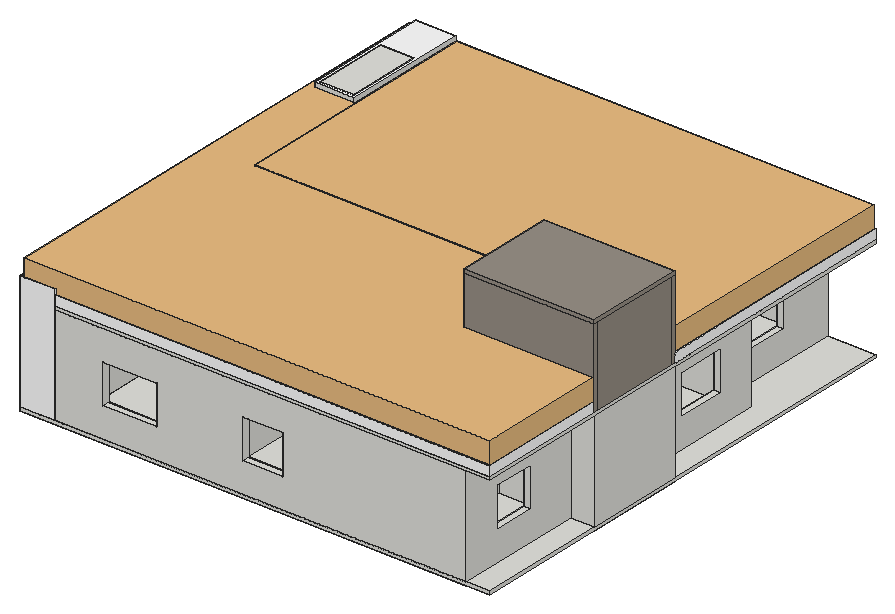
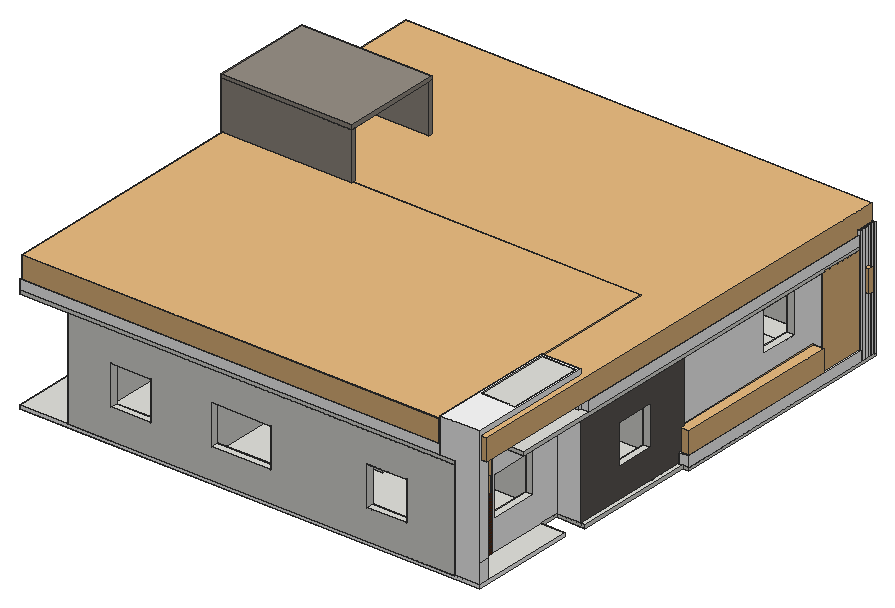
# SketchUp Ruby script. Lengths in inches.
U = 1.inch
M = Sketchup.active_model
def pt(a) = Geom::Point3d.new(a.map { |v| v * U })
def face(e, loops, mat)
  f = e.add_face(loops[0].map { |a| pt(a) })
  loops[1..].each { |l| e.add_face(l.map { |a| pt(a) }).erase! }
  f.material = f.back_material = mat if mat
  f
end
# faces: each face lists its corners as indices into pts; further lists are holes
def faces(e, pts, list, mat = nil) = list.each { |f| face(e, (f[0].is_a?(Array) ? f : [f]).map { |l| l.map { |i| pts[i] } }, mat) }
# xy, xz, yz: faces in a plane at the given z, y or x. An outline is a flat list of corners, or four numbers for a rectangle; further outlines are holes
def ring(l) = l.size == 4 ? [[l[0], l[1]], [l[2], l[1]], [l[2], l[3]], [l[0], l[3]]] : l.each_slice(2).to_a
def flat(e, list, mat, &to3) = list.each { |f| face(e, (f[0].is_a?(Array) ? f : [f]).map { |l| ring(l).map { |u, v| to3.(u, v) } }, mat) }
def xy(e, z, list, mat = nil) = flat(e, list, mat) { |x, y| [x, y, z] }
def xz(e, y, list, mat = nil) = flat(e, list, mat) { |x, z| [x, y, z] }
def yz(e, x, list, mat = nil) = flat(e, list, mat) { |y, z| [x, y, z] }
def lines(e, pts, list) = list.each { |a, b| e.add_line(pt(pts[a]), pt(pts[b])) }
# prism: a flat outline (further loops are holes) pulled along v
def prism(e, loops, v, mat = nil)
  f = face(e, loops, mat); d = Geom::Vector3d.new(v.map { |x| x * U })
  f.pushpull(f.normal.samedirection?(d) ? d.length : -d.length)
end
def box(e, o, s, mat = nil) = prism(e, [[o, [o[0] + s[0], o[1], o[2]], [o[0] + s[0], o[1] + s[1], o[2]], [o[0], o[1] + s[1], o[2]]]], [0, 0, s[2]], mat)
def at(x, y, z, deg = 0) = Geom::Transformation.translation(pt([x, y, z])) * Geom::Transformation.rotation(ORIGIN, Z_AXIS, deg.degrees)
def axes(o, x, y, z) = Geom::Transformation.new([*x, 0, *y, 0, *z, 0, *pt(o).to_a, 1])
def part(name) = M.definitions.add(name)
# library, detail: a bought-in or finely detailed component or shape, given as its bounding box
def library(name, o, s) = part(name).tap { |d| box(d.entities, o, s) }
def detail(e, o, s) = box(e.add_group.entities, o, s)
def put(e, d, t, mat = nil) = e.add_instance(d, t).tap { |i| i.material = mat if mat }
def group(e, t, mat = nil) = e.add_group.tap { |g| g.transformation = t; g.material = mat if mat }.entities
root = M.entities
M.materials.add("Bricks A03 100cm").color = [95, 90, 86]
M.materials.add("Manhattan Creative Coating MD 1125B 26.44cm").color = [255, 255, 255]
M.materials.add("Paint White Matte 002 0.02cm").color = [255, 255, 255]
M.materials.add("Pp-1846-msg 17.72cm").color = [255, 255, 255]
M.materials.add("Tiles L02 200cm").color = [152, 144, 134]
M.materials.add("Wintan - wpa36452 29.79cm").color = [255, 255, 255]
M.materials.add("Wood Mahogany 33-46 100cm").color = [84, 42, 21]
c1 = part("Stair tread")
box(c1.entities,[0,0,0],[9.89,48,7])
c2 = part("Group\#5")
box(c2.entities,[108.84,0,77],[43.96,112.5,7])
xy(c2.entities,124,[[49.47,0,59.37,48]])
xz(c2.entities,48,[[49.47,119,59.37,124]])
yz(c2.entities,49.47,[[0,119,48,124]])
put(c2.entities,c1,at(9.89,64.5,7))
put(c2.entities,c1,at(19.79,64.5,14))
put(c2.entities,c1,at(0,64.5,0))
put(c2.entities,c1,at(29.68,64.5,21))
put(c2.entities,c1,at(39.58,64.5,28))
put(c2.entities,c1,at(49.47,64.5,35))
put(c2.entities,c1,at(89.05,64.5,63))
put(c2.entities,c1,at(89.05,0,91))
put(c2.entities,c1,at(79.16,0,98))
put(c2.entities,c1,at(98.95,64.5,70))
put(c2.entities,c1,at(69.26,0,105))
put(c2.entities,c1,at(79.16,64.5,56))
put(c2.entities,c1,at(59.37,64.5,42))
put(c2.entities,c1,at(69.26,64.5,49))
put(c2.entities,c1,at(98.95,0,84))
put(c2.entities,c1,at(59.37,0,112))
c3 = part("Group\#20")
box(c3.entities,[0,0,0],[42,1.86,142.0625])
c4 = library("Group\#25",[0,0,0],[12.54,203.26,25.98])
c5 = library("Group1092\#1",[0.29,0.28,0],[3.28,6.3,0.11])
c6 = library("Group\#37",[0,0,0],[10.9375,10.44,50.62])
c7 = library("Spot Light",[-5.1,-5.1,-11.05],[10.2,10.2,11.05])
c8 = library("Group\#28",[0,0,0],[504.45,305.04,26.59])
c9 = library("Group\#27",[0,0,0],[563.06,581.04,25.98])
c10 = part("Component\#3")
xy(c10.entities,-1.4375,[[-40.6,0,0,4.4375]],"Wood Mahogany 33-46 100cm")
xy(c10.entities,3.0625,[[-40.6,0,0,4.4375]],"Wood Mahogany 33-46 100cm")
xz(c10.entities,0,[[-40.6,-1.4375,0,3.0625]],"Wood Mahogany 33-46 100cm")
xz(c10.entities,4.4375,[[-40.6,-1.4375,0,3.0625]],"Wood Mahogany 33-46 100cm")
yz(c10.entities,-40.6,[[0,-1.4375,4.4375,3.0625]],"Wood Mahogany 33-46 100cm")
yz(c10.entities,0,[[0,-1.4375,4.4375,3.0625]])
xy(root,102,[[178.31,333.5,187.31,362.5]])
xy(root,119,[[596.78,291,606.68,339]])
xy(root,120,[[[178.31,129,676.31,129,676.31,287.13,704.78,287.13,704.78,408.16,676.31,408.16,676.31,513.9,667.31,513.9,667.31,403.5,700.11,403.5,700.11,291,258.31,291,258.31,367.5,187.31,367.5,187.31,403.63,313.31,403.63,313.31,550.5,304.31,550.5,304.31,412.5,157.31,412.5,157.31,550.5,392.57,550.5,392.57,664.25,364.31,664.25,364.31,703.5,502.31,703.5,502.31,403.5,667.31,403.5,667.31,412.5,592.97,412.5,592.97,447.375,587.97,447.375,587.97,412.5,511.31,412.5,511.31,550.5,667.31,550.5,667.31,513.9,676.31,513.9,676.31,559.5,646.31,559.5,646.31,712.5,178.31,712.5,178.31,559.5,148.31,559.5,148.31,403.63,178.31,403.63],[187.31,559.5,187.31,703.5,355.31,703.5,355.31,660.44,383.57,660.44,383.57,600.44,355.31,600.44,355.31,595.72,383.57,595.72,383.57,559.5],[187.31,138,355.31,282],[511.31,138,511.31,282,587.97,282,587.97,247.1,592.97,247.1,592.97,282,667.31,282,667.31,138],[364.31,138,502.31,282],[511.31,559.5,637.31,703.5],[187.31,287,187.31,362.5,253.31,362.5,253.31,291,223.31,291,223.31,287]]])
xy(root,124,[[178.31,129,178.31,199.58,187.31,199.58,187.31,138,236.56,138,236.56,129],[236.56,129,302.56,138],[302.56,129,302.56,138,502.31,138,502.31,282,481.31,282,481.31,291,511.31,291,511.31,138,667.31,138,667.31,175.67,676.31,175.67,676.31,129],[273.14,138,273.21,138,273.27,138.01,273.34,138.02,273.4,138.03,273.46,138.05,273.52,138.08,273.58,138.1,273.64,138.13,273.7,138.17,273.85,138.29,273.97,138.44,274.01,138.5,274.04,138.56,274.0625,138.62,274.09,138.68,274.11,138.74,274.12,138.8,274.13,138.87,274.14,138.93,274.14,167.08,274.13,167.17,274.09,167.35,274.07,167.4375,274.04,167.52,273.96,167.68,273.86,167.84,273.8,167.91,273.74,167.97,273.68,168.04,273.61,168.1,273.53,168.15,273.46,168.2,273.38,168.25,273.3,168.28,273.21,168.32,273.13,168.35,272.95,168.39,272.86,168.4,272.59,168.4,272.5,168.39,272.32,168.35,272.24,168.32,272.15,168.28,272.07,168.25,271.91,168.15,271.84,168.1,271.77,168.04,271.71,167.97,271.65,167.91,271.59,167.84,271.49,167.68,271.41,167.52,271.38,167.4375,271.35,167.35,271.33,167.26,271.32,167.17,271.3125,167.08,271.31,166.99,216.79,166.99,216.79,204.56,216.98,204.5625,217.17,204.58,217.36,204.61,217.55,204.65,217.73,204.71,218.09,204.85,218.26,204.94,218.42,205.04,218.58,205.15,218.73,205.27,218.875,205.4,219.01,205.54,219.13,205.6875,219.25,205.84,219.35,206,219.45,206.17,219.53,206.34,219.6,206.52,219.66,206.7,219.71,206.89,219.75,207.08,219.77,207.27,219.78,207.46,219.78,207.65,219.77,207.84,219.75,208.04,219.71,208.22,219.66,208.41,219.6,208.59,219.53,208.77,219.45,208.94,219.35,209.11,219.25,209.27,219.13,209.43,219.01,209.57,218.875,209.71,218.73,209.84,218.58,209.96,218.42,210.07,218.26,210.17,218.09,210.26,217.91,210.34,217.55,210.46,217.36,210.5,217.17,210.53,216.98,210.55,216.79,210.56,216.79,248.125,271.31,248.125,271.3125,248.03,271.32,247.94,271.33,247.85,271.35,247.76,271.38,247.68,271.41,247.59,271.49,247.43,271.54,247.35,271.59,247.28,271.71,247.14,271.77,247.08,271.91,246.96,271.99,246.91,272.15,246.83,272.24,246.79,272.32,246.77,272.41,246.74,272.5,246.73,272.59,246.71,272.86,246.71,272.95,246.73,273.04,246.74,273.13,246.77,273.21,246.79,273.3,246.83,273.46,246.91,273.53,246.96,273.61,247.02,273.68,247.08,273.74,247.14,273.86,247.28,273.91,247.35,273.96,247.43,274.04,247.59,274.07,247.68,274.09,247.76,274.13,247.94,274.14,248.03,274.14,281.07,274.13,281.13,274.12,281.2,274.11,281.26,274.09,281.32,274.0625,281.38,274.04,281.44,274.01,281.5,273.97,281.56,273.85,281.71,273.7,281.83,273.64,281.87,273.58,281.9,273.52,281.92,273.46,281.95,273.4,281.97,273.34,281.98,273.27,281.99,273.21,282,273.14,282,355.31,282,355.31,174,364.31,174,364.31,138],[645.22,168.15,654.6,182.11,654.6,176.02,665.48,176.02,665.48,195.21,655.11,195.21,655.11,199.87,665.48,199.87,665.48,219.06,655.11,219.06,655.11,226.15,667.17,226.15,667.17,168.15],
  [355.31,174,355.31,291,334.31,286.5,313.31,291,400.31,291,400.31,287,403.31,287,403.31,286,400.31,286,400.31,282,364.31,282,364.31,174],[667.31,175.67,676.31,226.67],[654.6,182.11,654.6,182.86,655.11,182.86],[640.18,182.86,640.02,183.42,639.96,183.66,640.32,183.29,640.74,182.86],[654.6,182.86,655.11,195.21],
  [639.96,183.66,639.8,183.82,639.73,183.99,639.51,184.55,639.29,185.12,639.06,185.6875,638.83,186.25,638.6,186.82,638.37,187.38,637.89,188.5,637.14,190.15,636.88,190.68,636.61,191.22,636.34,191.74,636.0625,192.26,635.78,192.77,635.18,193.77,634.875,194.25,634.56,194.72,634.23,195.18,633.89,195.63,633.55,196.07,633.19,196.49,632.83,196.9,632.45,197.3,632.0625,197.68,631.66,198.05,631.25,198.4,630.83,198.74,630.39,199.06,629.9375,199.36,629.47,199.64,628.99,199.9,628.5,200.15,627.99,200.37,627.47,200.57,626.93,200.76,626.38,200.93,625.82,201.08,625.25,201.22,624.68,201.35,623.52,201.59,622.94,201.7,622.36,201.8,621.22,202.02,620.65,202.14,620.1,202.26,619.55,202.39,619.02,202.53,618.51,202.6875,618.01,202.86,617.53,203.04,617.07,203.25,616.63,203.47,616.22,203.72,615.83,203.99,615.46,204.29,615.11,204.6,614.79,204.94,614.49,205.29,614.21,205.67,613.94,206.0625,613.7,206.47,613.48,206.91,613.27,207.36,613.08,207.82,612.91,208.3,612.76,208.8,612.62,209.3125,612.5,209.84,612.39,210.38,612.3,210.94,612.22,211.51,612.15,212.09,612.09,212.68,612.05,213.29,612.02,213.9,611.99,214.53,611.98,215.16,611.98,215.8,611.99,216.46,612,217.11,612.02,217.78,612.05,218.46,612.13,219.82,612.17,220.51,612.23,221.21,612.28,221.91,612.34,222.61,612.4,223.32,612.47,224.02,612.53,224.73,612.67,226.15,616.25,226.15,616.22,225.53,616.1,223.64,616.01,221.78,615.99,221.16,615.97,220.55,615.95,219.9375,615.94,219.33,615.94,218.14,615.95,217.55,615.99,216.39,616.03,215.82,616.07,215.26,616.125,214.7,616.1875,214.15,616.26,213.62,616.34,213.09,616.4375,212.57,616.55,212.06,616.67,211.56,616.8,211.07,616.95,210.59,617.11,210.125,617.29,209.67,617.49,209.23,617.69,208.8,617.92,208.39,618.16,207.98,618.42,207.6,618.7,207.22,619,206.87,619.32,206.52,619.65,206.2,620.01,205.89,620.39,205.6,620.78,205.32,621.2,205.06,621.63,204.81,622.08,204.57,623.02,204.13,623.51,203.92,624,203.72,625,203.32,626.02,202.93,627.55,202.33,628.05,202.12,628.54,201.9,629.03,201.67,629.5,201.43,629.96,201.18,630.41,200.92,630.85,200.64,631.27,200.35,631.67,200.04,632.07,199.72,632.45,199.38,632.8125,199.04,633.17,198.68,633.51,198.31,633.84,197.92,634.16,197.53,634.47,197.12,634.76,196.71,635.05,196.28,635.33,195.84,635.6,195.4,635.86,194.94,636.11,194.48,636.35,194.01,636.58,193.53,636.81,193.04,637.03,192.55,637.24,192.05,637.45,191.54,637.65,191.03,637.84,190.51,638.03,189.98,638.39,188.92,638.57,188.38,638.91,187.3,639.07,186.75,639.24,186.2,639.4,185.64,639.56,185.09,639.71,184.53,639.87,183.98],[178.31,199.58,187.31,247.58],[654.6,199.87,655.11,219.06],[667.31,226.67,667.31,291,700.11,291,700.11,403.5,667.31,403.5,667.31,453.9,676.31,453.9,676.31,408.16,704.78,408.16,704.78,287.13,676.31,287.13,676.31,226.67],[178.31,247.58,178.31,333.5,187.31,333.5,187.31,287,223.31,287,223.31,291,253.31,291,253.31,330.63,258.31,330.63,258.31,291,313.31,291,313.31,282,187.31,282,187.31,247.58],
  [666.73,259.11,666.58,259.16,666.52,259.2,666.5,259.22,666.47,259.24,666.43,259.28,666.41,259.31,666.39,259.33,666.37,259.36,666.36,259.39,666.34,259.42,666.32,259.48,666.32,259.51,666.3125,259.54,666.31,259.58,666.31,269.45,667.31,269.45,667.31,259.58,667.3,259.54,667.3,259.51,667.26,259.39,667.24,259.36,667.23,259.33,667.21,259.31,667.1875,259.28,667.17,259.26,667.14,259.24,667.12,259.22,667.09,259.2,667.07,259.18,667.04,259.16,666.89,259.11],[666.31,269.45,666.31,277.78,666.3125,277.81,666.32,277.84,666.32,277.87,666.34,277.93,666.36,277.96,666.37,277.99,666.39,278.02,666.41,278.04,666.43,278.07,666.45,278.09,666.47,278.12,666.5,278.14,666.52,278.16,666.55,278.17,666.58,278.1875,666.61,278.2,666.64,278.22,666.67,278.23,666.7,278.23,666.73,278.24,666.76,278.24,666.79,278.25,666.82,278.25,666.86,278.24,666.89,278.24,666.92,278.23,666.95,278.23,666.98,278.22,667.01,278.2,667.04,278.1875,667.07,278.17,667.09,278.16,667.12,278.14,667.17,278.09,667.1875,278.07,667.21,278.04,667.23,278.02,667.24,277.99,667.26,277.96,667.3,277.84,667.3,277.81,667.31,277.78,667.31,269.45],[313.31,282,313.31,291,334.31,286.5],[313.31,282,334.31,286.5,355.31,282],[355.31,282,334.31,286.5,355.31,291],
  [400.31,282,403.31,286],[403.31,282,451.31,291],[451.31,282,451.31,291,454.31,291,454.31,287,478.31,287,478.31,291,481.31,291,481.31,282,478.31,282,478.31,286,454.31,286,454.31,282],[454.31,282,478.31,286],[400.31,287,403.31,291],
  [454.31,287,478.31,291],[304.31,291,304.31,403.5,304.43,401.96,304.43,292.54],[304.31,291,304.43,292.54,304.43,291],[304.43,291,304.43,292.54,308.81,347.25,313.31,291],[313.31,291,308.81,347.25,313.31,403.5],
  [502.31,291,502.31,291.22,502.33,291.22],[502.31,291,502.33,291.22,511.29,291.22,511.31,291],[511.31,291,511.29,291.22,511.31,291.22],[502.31,291.22,502.31,403.5,506.81,347.25,502.33,291.22],[502.33,291.22,506.81,347.25,511.29,291.22],
  [511.29,291.22,506.81,347.25,511.31,403.5,511.31,291.22],[511.31,291.22,511.37,550.5],[304.43,292.54,304.43,401.96,308.81,347.25],[178.31,333.5,178.31,367.5,258.31,367.5,258.31,362.5,187.31,362.5,187.31,333.5],[308.81,347.25,304.43,401.96,304.43,403.5,313.31,403.5],
  [506.81,347.25,502.31,403.5,511.31,403.5],[482.12,382.5,502.31,449.24],[304.43,401.96,304.31,403.5,304.31,403.63,304.43,403.63],[304.43,403.5,313.31,403.63],[547.31,403.5,547.31,412.5,587.97,412.5,587.97,447.375,592.97,447.375,592.97,412.5,667.31,412.5,667.31,403.5],
  [148.31,403.63,148.31,454.3,157.31,454.3,157.31,412.5,268.31,412.5,268.31,403.63],[268.31,403.63,268.43,412.5],[645.22,465.17,654.6,479.125,654.6,473.03,665.48,473.03,665.48,492.22,655.11,492.22,655.11,496.88,665.48,496.88,665.48,516.07,655.11,516.07,655.11,523.17,667.17,523.17,667.17,465.17],[654.6,479.125,654.6,479.87,655.11,479.87],[640.18,479.87,640.02,480.43,639.96,480.67,640.32,480.3,640.74,479.87],
  [654.6,479.87,655.11,492.22],[639.96,480.67,639.9,480.74,639.8,480.84,639.73,481,639.51,481.57,639.29,482.13,638.83,483.27,638.6,483.83,638.37,484.4,638.13,484.96,637.89,485.51,637.64,486.07,637.39,486.62,637.14,487.16,636.88,487.7,636.34,488.76,636.0625,489.27,635.78,489.78,635.48,490.29,635.18,490.78,634.875,491.26,634.56,491.73,634.23,492.2,633.89,492.65,633.55,493.08,633.19,493.51,632.83,493.92,632.45,494.32,632.0625,494.7,631.66,495.07,631.25,495.42,630.83,495.75,630.39,496.07,629.9375,496.37,629.47,496.65,628.99,496.92,628.5,497.16,627.99,497.38,627.47,497.59,626.93,497.77,626.38,497.94,625.82,498.09,625.25,498.23,624.68,498.36,623.52,498.6,622.36,498.82,620.65,499.15,619.55,499.41,619.02,499.55,618.51,499.7,618.01,499.87,617.53,500.06,617.07,500.26,616.63,500.49,616.22,500.73,615.83,501.01,615.46,501.3,615.11,501.61,614.79,501.95,614.49,502.31,614.21,502.68,613.94,503.08,613.7,503.49,613.48,503.92,613.27,504.37,613.08,504.84,612.91,505.32,612.76,505.82,612.62,506.33,612.5,506.86,612.39,507.4,612.3,507.95,612.22,508.52,612.15,509.1,612.09,509.7,612.05,510.3,612.02,510.91,611.99,511.54,611.98,512.17,611.98,512.82,611.99,513.47,612,514.13,612.02,514.8,612.05,515.47,612.09,516.15,612.17,517.53,612.23,518.22,612.28,518.92,612.4,520.33,612.47,521.04,612.53,521.75,612.67,523.17,616.25,523.17,616.22,522.54,616.14,521.28,616.1,520.66,616.07,520.03,616.01,518.79,615.99,518.18,615.97,517.5625,615.95,516.95,615.94,516.35,615.94,515.15,615.95,514.5625,615.97,513.98,615.99,513.4,616.03,512.83,616.07,512.27,616.125,511.71,616.1875,511.17,616.26,510.63,616.34,510.1,616.4375,509.58,616.55,509.07,616.67,508.57,616.8,508.08,616.95,507.6,617.11,507.14,617.29,506.68,617.49,506.24,617.69,505.81,617.92,505.4,618.16,505,618.42,504.61,618.7,504.24,619,503.88,619.32,503.54,619.65,503.21,620.01,502.9,620.39,502.61,620.78,502.33,621.2,502.07,621.63,501.82,622.08,501.59,622.55,501.36,623.02,501.14,623.51,500.94,624,500.73,624.5,500.53,625,500.34,625.51,500.14,626.02,499.95,627.04,499.55,627.55,499.34,628.05,499.13,628.54,498.91,629.03,498.6875,629.5,498.45,629.96,498.2,630.41,497.93,630.85,497.65,631.27,497.36,631.67,497.05,632.07,496.73,632.45,496.4,632.8125,496.05,633.17,495.69,633.51,495.32,633.84,494.9375,634.16,494.54,634.47,494.14,634.76,493.72,635.05,493.29,635.33,492.86,635.6,492.41,635.86,491.96,636.11,491.5,636.35,491.02,636.81,490.06,637.03,489.5625,637.24,489.0625,637.45,488.55,637.65,488.04,638.03,487,638.39,485.94,638.57,485.4,638.74,484.86,638.91,484.31,639.07,483.76,639.24,483.21,639.4,482.66,639.56,482.1,639.71,481.55,639.87,480.99],[654.6,496.88,655.11,516.07],[148.31,502.3,148.31,559.5,178.31,559.5,178.31,594.58,187.31,594.58,187.31,559.5,392.57,559.5,392.57,550.5,157.31,550.5,157.31,502.3],[392.57,550.5,502.31,559.5],
  [214.32,559.5,281.06,580.44],[637.31,586.67,646.31,646.67],[502.31,595.5,502.31,703.5,473.12,703.5,473.12,712.5,546.3125,712.5,546.3125,703.5,511.31,703.5,511.31,595.5],[355.31,595.72,355.31,600.44,383.57,600.44,383.57,660.44,355.31,660.44,355.31,703.5,284.58,703.5,284.58,712.5,401.12,712.5,401.12,703.5,364.31,703.5,364.31,664.25,392.57,664.25,392.57,595.72],[637.31,646.67,637.31,703.5,594.3125,703.5,594.3125,712.5,646.31,712.5,646.31,646.67],
  [178.31,654.58,178.31,712.5,236.58,712.5,236.58,703.5,187.31,703.5,187.31,654.58],[401.12,703.5,473.12,712.5]])
xy(root,160,[[236.56,129,302.56,138],[406.31,129,454.31,138],[667.31,175.67,676.31,226.67],[178.31,199.58,187.31,247.58],[667.31,453.9,676.31,513.9],
  [148.31,454.3,157.31,502.3],[637.31,586.67,646.31,646.67],[178.31,594.58,187.31,654.58],[236.58,703.5,284.58,712.5],[401.12,703.5,473.12,712.5],
  [546.3125,703.5,594.3125,712.5]])
xy(root,208,[[236.56,129,302.56,138],[406.31,129,454.31,138],[355.31,138,364.31,174],[667.31,175.67,676.31,226.67],[178.31,199.58,187.31,247.58],
  [403.31,282,451.31,291],[511.31,282,547.31,291],[253.31,330.63,258.31,362.5],[178.31,333.5,187.31,362.5],[178.31,367.5,187.31,403.63],
  [511.31,403.5,547.31,412.5],[268.31,403.63,304.31,412.5],[667.31,453.9,676.31,513.9],[148.31,454.3,157.31,502.3],[383.57,559.5,392.57,595.72],
  [502.31,559.5,511.31,595.5],[637.31,586.67,646.31,646.67],[178.31,594.58,187.31,654.58],[236.58,703.5,284.58,712.5],[401.12,703.5,473.12,712.5],
  [546.3125,703.5,594.3125,712.5]])
xy(root,226,[[178.31,333.5,187.31,362.5]])
xy(root,244,[[[178.31,129,676.31,129,676.31,287.13,704.78,287.13,704.78,408.16,676.31,408.16,676.31,513.9,667.31,513.9,667.31,403.5,700.11,403.5,700.11,291,258.31,291,258.31,367.5,187.31,367.5,187.31,403.63,313.31,403.63,313.31,550.5,304.31,550.5,304.31,412.5,157.31,412.5,157.31,550.5,392.57,550.5,392.57,664.25,364.31,664.25,364.31,703.5,502.31,703.5,502.31,403.5,667.31,403.5,667.31,412.5,592.97,412.5,592.97,447.375,587.97,447.375,587.97,412.5,511.31,412.5,511.31,550.5,667.31,550.5,667.31,513.9,676.31,513.9,676.31,559.5,646.31,559.5,646.31,712.5,178.31,712.5,178.31,559.5,148.31,559.5,148.31,403.63,178.31,403.63],[187.31,559.5,187.31,703.5,355.31,703.5,355.31,660.44,383.57,660.44,383.57,600.44,355.31,600.44,355.31,595.72,383.57,595.72,383.57,559.5],[187.31,138,355.31,282],[511.31,138,511.31,282,587.97,282,587.97,247.1,592.97,247.1,592.97,282,667.31,282,667.31,138],[364.31,138,502.31,282],[511.31,559.5,637.31,703.5],[187.31,287,187.31,362.5,253.31,362.5,253.31,291,223.31,291,223.31,287]]])
xy(root,290.9375,[[152.01,563.2,192.61,654.625]])
xz(root,129,[[[178.31,124,676.31,244],[236.56,160,302.56,208],[406.31,160,454.31,208]]])
xz(root,138,[[[187.31,124,187.31,244,355.31,244,355.31,208,364.31,208,364.31,244,502.31,244,502.31,124],[236.56,160,302.56,208],[406.31,160,454.31,208]],[511.31,124,667.31,244]])
xz(root,174,[[355.31,124,364.31,208]])
xz(root,175.67,[[667.31,160,676.31,208]])
xz(root,199.58,[[178.31,160,187.31,208]])
xz(root,226.67,[[667.31,160,676.31,208]])
xz(root,247.1,[[587.97,124,592.97,244]])
xz(root,247.58,[[178.31,160,187.31,208]])
xz(root,282,[[187.31,124,355.31,244],[364.31,124,403.31,124,403.31,208,451.31,208,451.31,124,502.31,124,502.31,244,364.31,244],[547.31,124,587.97,124,587.97,244,511.31,244,511.31,208,547.31,208],[592.97,124,667.31,244]])
xz(root,287,[[187.31,124,223.31,244]])
xz(root,287.13,[[676.31,124,704.78,244]])
xz(root,291,[[223.31,124,253.31,244],[258.31,124,258.31,244,700.11,244,700.11,124,547.31,124,547.31,208,511.31,208,511.31,124,451.31,124,451.31,208,403.31,208,403.31,124]])
xz(root,330.63,[[253.31,124,258.31,208]])
xz(root,333.5,[[178.31,208,187.31,226]])
xz(root,362.5,[[187.31,124,258.31,124,258.31,208,253.31,208,253.31,244,187.31,244,187.31,226,178.31,226,178.31,208,187.31,208]])
xz(root,367.5,[[178.31,124,178.31,208,187.31,208,187.31,244,258.31,244,258.31,124]])
xz(root,403.5,[[502.31,124,511.31,124,511.31,208,547.31,208,547.31,124,700.11,124,700.11,244,502.31,244]])
xz(root,403.63,[[148.31,124,268.31,124,268.31,208,304.31,208,304.31,124,313.31,124,313.31,244,187.31,244,187.31,208,178.31,208,178.31,244,148.31,244]],"Pp-1846-msg 17.72cm")
xz(root,408.16,[[676.31,124,704.78,244]])
xz(root,412.5,[[157.31,124,157.31,244,304.31,244,304.31,208,268.31,208,268.31,124],[547.31,124,547.31,208,511.31,208,511.31,244,587.97,244,587.97,124],[592.97,124,667.31,244]])
xz(root,447.375,[[587.97,124,592.97,244]])
xz(root,453.9,[[667.31,160,676.31,208]])
xz(root,454.3,[[148.31,160,157.31,208]])
xz(root,502.3,[[148.31,160,157.31,208]])
xz(root,513.9,[[667.31,160,676.31,208]])
xz(root,550.5,[[157.31,124,304.31,244],[304.31,124,313.31,244],[313.31,124,392.57,244],[511.31,124,511.37,244],[511.37,124,667.31,244]])
xz(root,559.5,[[187.31,124,187.31,244,383.57,244,383.57,208,392.57,208,392.57,124],[502.31,124,502.31,208,511.31,208,511.31,244,637.31,244,637.31,124],[646.31,124,676.31,244]])
xz(root,559.5,[[148.31,124,178.31,244]],"Pp-1846-msg 17.72cm")
xz(root,586.67,[[637.31,160,646.31,208]])
xz(root,594.58,[[178.31,160,187.31,208]])
xz(root,595.5,[[502.31,124,511.31,208]])
xz(root,595.72,[[355.31,124,392.57,124,392.57,208,383.57,208,383.57,244,355.31,244]])
xz(root,600.44,[[355.31,124,383.57,244]])
xz(root,646.67,[[637.31,160,646.31,208]])
xz(root,654.58,[[178.31,160,187.31,208]])
xz(root,660.44,[[355.31,124,383.57,244]])
xz(root,664.25,[[364.31,124,392.57,244]])
xz(root,703.5,[[[187.31,124,355.31,244],[236.58,160,284.58,208]],[[364.31,124,502.31,244],[401.12,160,473.12,208]],[511.31,124,546.3125,244],[546.3125,124,594.3125,160],[594.3125,124,637.31,124,637.31,244,546.3125,244,546.3125,208,594.3125,208]])
xz(root,712.5,[[[178.31,124,646.31,244],[401.12,160,473.12,208],[236.58,160,284.58,208],[546.3125,160,594.3125,208]]])
yz(root,148.31,[[[403.63,124,559.5,244],[454.3,160,502.3,208]]],"Bricks A03 100cm")
yz(root,157.31,[[412.5,124,454.3,124,454.3,208,502.3,208,502.3,160,454.3,160,454.3,124,550.5,124,550.5,244,412.5,244]])
yz(root,178.31,[[700.5,124,712.5,244]])
yz(root,178.31,[[[129,124,129,244,403.63,244,403.63,208,367.5,208,367.5,124],[199.58,160,247.58,208],[333.5,208,362.5,226]],[[559.5,124,700.5,244],[594.58,160,654.58,208]]],"Pp-1846-msg 17.72cm")
yz(root,187.31,[[[138,124,282,244],[199.58,160,247.58,208]],[287,124,362.5,124,362.5,208,333.5,208,333.5,226,362.5,226,362.5,244,287,244],[[559.5,124,703.5,244],[594.58,160,654.58,208]],[367.5,208,403.63,244]])
yz(root,223.31,[[287,124,291,244]])
yz(root,236.56,[[129,160,138,208]])
yz(root,236.58,[[703.5,160,712.5,208]])
yz(root,253.31,[[291,124,319.5,244],[319.5,124,319.5,244,362.5,244,362.5,208,330.63,208,330.63,124]])
yz(root,258.31,[[291,124,330.63,124,330.63,208,362.5,208,362.5,124,367.5,124,367.5,244,291,244]])
yz(root,268.31,[[403.63,124,412.5,208]])
yz(root,284.58,[[703.5,160,712.5,208]])
yz(root,302.56,[[129,160,138,208]])
yz(root,304.31,[[403.63,124,403.63,208,412.5,208,412.5,244,550.5,244,550.5,124]])
yz(root,313.31,[[403.63,124,550.5,244]])
yz(root,355.31,[[174,124,174,208,138,208,138,244,282,244,282,124],[595.72,124,600.44,244],[660.44,124,703.5,244]])
yz(root,364.31,[[174,124,282,124,282,244,138,244,138,208,174,208],[664.25,124,703.5,244]])
yz(root,383.57,[[600.44,124,660.44,244],[559.5,208,595.72,244]])
yz(root,392.57,[[550.5,124,559.5,124,559.5,208,595.72,208,595.72,124,664.25,124,664.25,244,550.5,244]])
yz(root,401.12,[[703.5,160,712.5,208]])
yz(root,403.31,[[282,124,291,208]])
yz(root,406.31,[[129,160,138,208]])
yz(root,451.31,[[282,124,291,208]])
yz(root,454.31,[[129,160,138,208]])
yz(root,473.12,[[703.5,160,712.5,208]])
yz(root,502.31,[[138,124,282,244],[403.5,124,403.5,244,703.5,244,703.5,124,595.5,124,595.5,208,559.5,208,559.5,124]])
yz(root,511.31,[[138,124,291,124,291,208,282,208,282,244,138,244],[403.5,124,550.5,124,550.5,244,412.5,244,412.5,208,403.5,208],[595.5,124,703.5,124,703.5,244,559.5,244,559.5,208,595.5,208]])
yz(root,546.3125,[[703.5,160,712.5,208]])
yz(root,547.31,[[282,124,291,208],[403.5,124,412.5,208]])
yz(root,587.97,[[247.1,124,282,244],[412.5,124,447.375,244]])
yz(root,592.97,[[247.1,124,282,244],[412.5,124,424.8,244],[424.8,124,437.1,244],[437.1,124,447.375,244]])
yz(root,594.3125,[[703.5,160,712.5,208]])
yz(root,637.31,[[[559.5,124,703.5,244],[586.67,160,646.67,208]]])
yz(root,646.31,[[[559.5,124,712.5,244],[586.67,160,646.67,208]]])
yz(root,667.31,[[[138,124,282,244],[175.67,160,226.67,208]],[412.5,124,412.5,244,513.9,244,513.9,208,453.9,208,453.9,160,513.9,160,513.9,244,550.5,244,550.5,124]])
yz(root,676.31,[[[129,124,287.13,244],[175.67,160,226.67,208]],[[408.16,124,559.5,244],[453.9,160,513.9,208]]])
yz(root,700.11,[[291,124,403.5,244]])
yz(root,704.78,[[287.13,124,408.16,244]])
g1 = group(root,at(148.31,129,120))
xy(g1,0,[[[-12,0,-12,283.19,-4.75,283.19,-4.75,430.5,30,430.5,30,454.5,0,454.5,0,583.5,556.47,583.5,556.47,0],[448.47,162,551.8,162,551.8,274.5,399,274.5,399,210,448.47,210]]],"Pp-1846-msg 17.72cm")
xy(g1,4,[[[-12,0,556.47,0,556.47,583.5,0,583.5,0,454.5,30,454.5,30,430.5,-4.75,430.5,-4.75,283.19,-12,283.19],[448.47,162,448.47,210,399,210,399,274.5,551.8,274.5,551.8,162]]])
xz(g1,0,[[-12,0,556.47,4]])
xz(g1,162,[[448.47,0,551.8,4]])
xz(g1,210,[[399,0,448.47,4]])
xz(g1,274.5,[[399,0,551.8,4]])
xz(g1,283.19,[[-12,0,-4.75,4]])
xz(g1,430.5,[[-4.75,0,0,4],[0,0,30,4]])
xz(g1,454.5,[[0,0,30,4]])
xz(g1,583.5,[[0,0,556.47,4]],"Pp-1846-msg 17.72cm")
yz(g1,-12,[[0,0,283.19,4]])
yz(g1,-4.75,[[283.19,0,430.5,4]])
yz(g1,0,[[454.5,0,583.5,4]],"Wintan - wpa36452 29.79cm")
yz(g1,30,[[430.5,0,454.5,4]])
yz(g1,399,[[210,0,274.5,4]])
yz(g1,448.47,[[162,0,210,4]])
yz(g1,551.8,[[162,0,274.5,4]])
yz(g1,556.47,[[0,0,583.5,4]])
g2 = group(root,at(547.31,291,124))
xz(g2,0,[[49.47,119,59.37,124]])
g3 = group(g2,at(0,0,0))
xy(g3,119,[[49.47,0,59.37,48]])
yz(g3,59.37,[[0,119,48,124]])
put(g3,c1,at(9.89,64.5,7))
put(g3,c2,at(0,0,0))
g4 = group(root,at(178.31,700.5,124))
xy(g4,0,[[-30,0,0,12]])
xy(g4,124,[[-30,-141,18,-137.3],[0,0,18,12]])
xy(g4,153.125,[[-30,-137.3,-30,-42.17,18,-42.17,18,-137.3,14.3,-137.3,14.3,-45.875,-26.3,-45.875,-26.3,-137.3],[-30,-42.17,18,0]])
xy(g4,166.9375,[[[-30,-141,18,12],[-26.3,-137.3,14.3,-45.875]]],"Paint White Matte 002 0.02cm")
xz(g4,-141,[[-30,124,18,166.9375]])
xz(g4,-137.3,[[-30,124,-30,153.125,-26.3,153.125,-26.3,166.9375,14.3,166.9375,14.3,153.125,18,153.125,18,124]],"Paint White Matte 002 0.02cm")
xz(g4,-45.875,[[-26.3,153.125,14.3,166.9375]])
xz(g4,0,[[-30,0,0,0,0,124,18,124,18,153.125,-30,153.125]])
xz(g4,12,[[-30,0,-30,166.9375,18,166.9375,18,124,0,124,0,0]],"Paint White Matte 002 0.02cm")
yz(g4,-30,[[0,24,0,153.125,-137.3,153.125,-137.3,124,-141,124,-141,166.9375,12,166.9375,12,24]],"Paint White Matte 002 0.02cm")
yz(g4,-30,[[0,0,12,24]],"Wintan - wpa36452 29.79cm")
yz(g4,-26.3,[[-137.3,153.125,-45.875,166.9375]])
yz(g4,0,[[0,0,12,124]])
yz(g4,14.3,[[-137.3,153.125,-45.875,166.9375]])
yz(g4,18,[[-141,124,-137.3,124,-137.3,153.125,0,153.125,0,124,12,124,12,166.9375,-141,166.9375]])
g5 = group(root,at(136.31,129,124),"Manhattan Creative Coating MD 1125B 26.44cm")
put(g5,c3,at(0,4.26,0))
put(g5,c3,at(0,8.53,0))
put(g5,c3,at(0,17.05,0))
put(g5,c3,at(0,21.3125,0))
put(g5,c3,at(0,12.79,0))
put(g5,c3,at(0,0,0))
g6 = group(root,at(136.31,152.17,124))
xy(g6,0,[[0,0,0,260.02,12,260.02,12,251.45,6.3125,251.45,6.3125,0]])
xy(g6,12,[[0,0,3,0,3,255.74,12,255.74,12,260.02,0,260.02],[3,0,6.3125,0,6.3125,251.45,12,251.45,12,255.74,3,255.74]])
xz(g6,0,[[0,0,6.3125,12]])
xz(g6,251.45,[[6.3125,0,12,12]])
xz(g6,260.02,[[0,0,12,12]],"Wintan - wpa36452 29.79cm")
yz(g6,0,[[0,0,260.02,12]],"Wintan - wpa36452 29.79cm")
yz(g6,6.3125,[[0,0,251.45,12]])
yz(g6,12,[[251.45,0,260.02,12]])
put(g6,c4,at(1.43,54.05,12))
g7 = group(root,at(177.31,658.33,124),"Wood Mahogany 33-46 100cm")
prism(g7,[[[1.05,0,0],[1.05,0,124],[21.17,0.02,124],[21.17,0.02,153.125],[0.05,0,153.125],[0.05,0,150.0625],[0.05,0,147],[0.05,0,143.9375],[0.05,0,140.875],[0.05,0,137.8125],[0.05,0,134.75],[0.05,0,131.6875],[0.05,0,128.625],[0.05,0,125.5625],[0.05,0,122.5],[0.05,0,119.4375],[0.05,0,116.375],[0.05,0,113.3125],[0.05,0,110.25],[0.05,0,107.1875],[0.05,0,104.125],[0.05,0,101.0625],[0.05,0,98],[0.05,0,94.9375],[0.05,0,91.875],[0.05,0,88.8125],[0.05,0,85.75],[0.05,0,82.6875],[0.05,0,79.625],[0.05,0,76.5625],[0.05,0,73.5],[0.05,0,70.4375],[0.05,0,67.375],[0.05,0,64.3125],[0.05,0,61.25],[0.05,0,58.1875],[0.05,0,55.125],[0.05,0,52.0625],[0.05,0,49],[0.05,0,45.9375],[0.05,0,42.875],[0.05,0,39.8125],[0.05,0,36.75],[0.05,0,33.6875],[0.05,0,30.625],[0.05,0,27.5625],[0.05,0,24.5],[0.05,0,21.4375],[0.05,0,18.375],[0.05,0,15.3125],[0.05,0,12.25],[0.05,0,9.1875],[0.05,0,6.125],[0.05,0,3.0625],[0.05,0,0]]],[-0.05,42.17,0],"Wood Mahogany 33-46 100cm")
put(root,c5,axes([140.75,210.13,131.41],[-0.00298,-16.24442,0.00298],[0,0.00314,17.09939],[-17.09939,0.00314,0]))
put(root,c6,axes([130.73,140.7,197.25],[0.5325,0,0],[0,0.5325,0],[0,0,0.5325]))
put(root,c7,axes([182.71,678.84,200.09],[-1,0,0],[0,1,0],[0,0,-1.72]))
put(root,c7,axes([171.96,678.84,219.1],[1,0,0],[0,1,0],[0,0,1.72]))
put(root,c7,axes([171.96,678.84,219.1],[-1,0,0],[0,1,0],[0,0,1.72]))
put(root,c6,at(166.86,673.5,200.09))
g8 = group(root,at(148.31,129,244))
prism(g8,[[[-9.4375,23.17,0],[-9.4375,529.33,0],[30.05,529.33,0],[30.05,583.5,0],[556.47,583.5,0],[556.47,0,0],[30,0,0],[30,23.17,0]],[[551.8,274.5,0],[399,274.5,0],[399,210,0],[448.47,210,0],[448.47,162,0],[551.8,162,0]]],[0,0,4])
g9 = group(root,at(547.31,286.5,248),"Tiles L02 200cm")
g10 = group(g9,at(0,0,96))
box(g10,[0,0,0],[157.47,121.5,4.5])
g11 = group(g9,at(0,0,0))
box(g11,[0,0,0],[157.47,4.5,96])
g12 = group(g9,at(152.8,4.5,0))
box(g12,[0,0,0],[4.67,112.5,96])
g13 = group(g9,at(0,117,0))
box(g13,[0,0,0],[157.47,4.5,96])
g14 = group(root,at(138.87,129,248),"Wintan - wpa36452 29.79cm")
xy(g14,0,[[39.4375,0,39.4375,23.17,45.4375,23.17,45.4375,6,565.91,6,565.91,0],[0,23.17,0,430.5,57.4375,430.5,57.4375,583.5,565.91,583.5,565.91,279,559.91,279,559.91,577.5,63.4375,577.5,63.4375,424.5,6,424.5,6,29.17,45.4375,29.17,45.4375,23.17]])
xy(g14,12,[[39.4375,0,565.91,0,565.91,157.5,562.91,157.5,562.91,3,42.4375,3,42.4375,26.17,3,26.17,3,427.5,60.4375,427.5,60.4375,580.5,562.91,580.5,562.91,279,565.91,279,565.91,583.5,57.4375,583.5,57.4375,430.5,0,430.5,0,23.17,39.4375,23.17],[42.4375,3,562.91,3,562.91,157.5,559.91,157.5,559.91,6,45.4375,6,45.4375,29.17,6,29.17,6,424.5,63.4375,424.5,63.4375,577.5,559.91,577.5,559.91,279,562.91,279,562.91,580.5,60.4375,580.5,60.4375,427.5,3,427.5,3,26.17,42.4375,26.17]])
xz(g14,0,[[39.4375,0,565.91,12]])
xz(g14,6,[[45.4375,0,559.91,12]])
xz(g14,23.17,[[0,0,39.4375,12]])
xz(g14,29.17,[[6,0,45.4375,12]])
xz(g14,157.5,[[559.91,0,565.91,12]])
xz(g14,279,[[559.91,0,565.91,12]])
xz(g14,424.5,[[6,0,63.4375,12]])
xz(g14,430.5,[[0,0,57.4375,12]])
xz(g14,577.5,[[63.4375,0,559.91,12]])
xz(g14,583.5,[[57.4375,0,565.91,12]])
yz(g14,0,[[23.17,0,430.5,12]])
yz(g14,6,[[29.17,0,424.5,12]])
yz(g14,39.4375,[[0,0,23.17,12]])
yz(g14,45.4375,[[6,0,29.17,12]])
yz(g14,57.4375,[[430.5,0,583.5,12]])
yz(g14,63.4375,[[424.5,0,577.5,12]])
yz(g14,559.91,[[6,0,157.5,12],[279,0,577.5,12]])
yz(g14,565.91,[[0,0,157.5,12],[279,0,583.5,12]])
put(root,c8,at(198.91,406.03,260))
put(root,c9,at(140.3,130.43,260))
put(root,c10,at(192.61,647.55,277.125))
put(root,c10,at(192.61,631.15,277.125))
put(root,c10,at(192.61,614.75,277.125))
put(root,c10,at(192.61,598.35,277.125))
put(root,c10,at(192.61,581.95,277.125))
put(root,c10,at(192.61,565.55,277.125))
